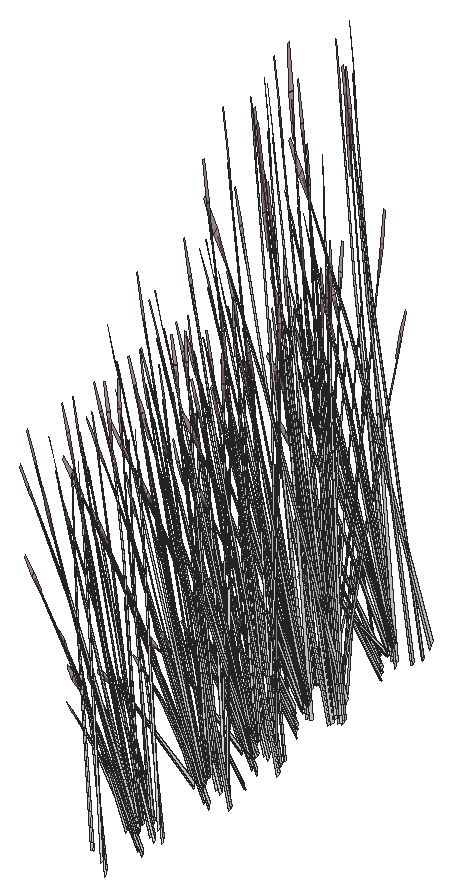
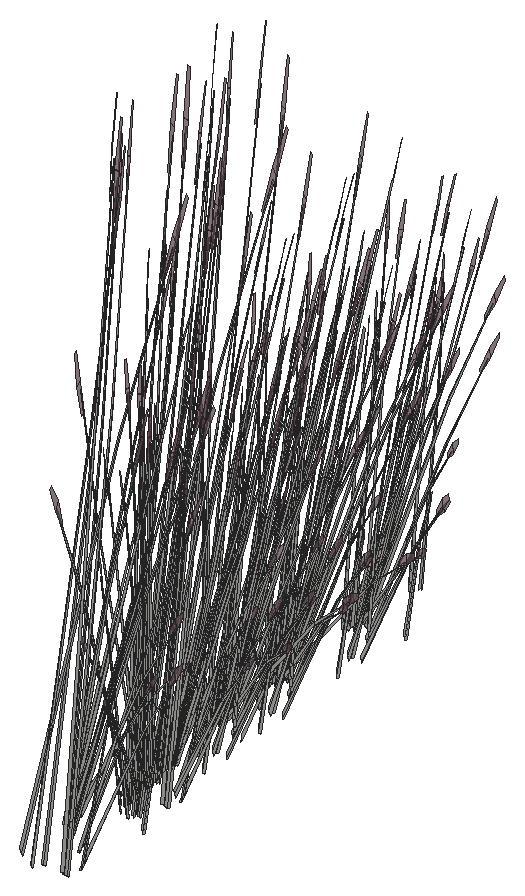
# SketchUp Ruby script. Lengths in inches.
U = 1.inch
M = Sketchup.active_model
def pt(a) = Geom::Point3d.new(a.map { |v| v * U })
def face(e, loops, mat)
  f = e.add_face(loops[0].map { |a| pt(a) })
  loops[1..].each { |l| e.add_face(l.map { |a| pt(a) }).erase! }
  f.material = f.back_material = mat if mat
  f
end
# faces: each face lists its corners as indices into pts; further lists are holes
def faces(e, pts, list, mat = nil) = list.each { |f| face(e, (f[0].is_a?(Array) ? f : [f]).map { |l| l.map { |i| pts[i] } }, mat) }
# xy, xz, yz: faces in a plane at the given z, y or x. An outline is a flat list of corners, or four numbers for a rectangle; further outlines are holes
def ring(l) = l.size == 4 ? [[l[0], l[1]], [l[2], l[1]], [l[2], l[3]], [l[0], l[3]]] : l.each_slice(2).to_a
def flat(e, list, mat, &to3) = list.each { |f| face(e, (f[0].is_a?(Array) ? f : [f]).map { |l| ring(l).map { |u, v| to3.(u, v) } }, mat) }
def xy(e, z, list, mat = nil) = flat(e, list, mat) { |x, y| [x, y, z] }
def xz(e, y, list, mat = nil) = flat(e, list, mat) { |x, z| [x, y, z] }
def yz(e, x, list, mat = nil) = flat(e, list, mat) { |y, z| [x, y, z] }
def lines(e, pts, list) = list.each { |a, b| e.add_line(pt(pts[a]), pt(pts[b])) }
# prism: a flat outline (further loops are holes) pulled along v
def prism(e, loops, v, mat = nil)
  f = face(e, loops, mat); d = Geom::Vector3d.new(v.map { |x| x * U })
  f.pushpull(f.normal.samedirection?(d) ? d.length : -d.length)
end
def box(e, o, s, mat = nil) = prism(e, [[o, [o[0] + s[0], o[1], o[2]], [o[0] + s[0], o[1] + s[1], o[2]], [o[0], o[1] + s[1], o[2]]]], [0, 0, s[2]], mat)
def at(x, y, z, deg = 0) = Geom::Transformation.translation(pt([x, y, z])) * Geom::Transformation.rotation(ORIGIN, Z_AXIS, deg.degrees)
def axes(o, x, y, z) = Geom::Transformation.new([*x, 0, *y, 0, *z, 0, *pt(o).to_a, 1])
def part(name) = M.definitions.add(name)
# library, detail: a bought-in or finely detailed component or shape, given as its bounding box
def library(name, o, s) = part(name).tap { |d| box(d.entities, o, s) }
def detail(e, o, s) = box(e.add_group.entities, o, s)
def put(e, d, t, mat = nil) = e.add_instance(d, t).tap { |i| i.material = mat if mat }
def group(e, t, mat = nil) = e.add_group.tap { |g| g.transformation = t; g.material = mat if mat }.entities
root = M.entities
M.materials.add("LightPink_Translucent").color = [144, 107, 117]
M.materials["LightPink_Translucent"].alpha = 0.75
c1 = part("blade")
p = [[2.15,0.21,22],[0,0.17,0],[0.09,0.45,0],[2.18,0.31,22],[2.29,0.31,22],[0.38,0.45,0],
  [2.48,0.24,33],[2.49,0.24,33],[2.48,0.22,33]]
faces(c1.entities,p,[[0,1,2,3],[4,5,2,3],[6,3,4,7],[8,0,3,6]])
c2 = part("seeds")
p = [[0.3,-0.1,1.38],[-0.01,-0.03,1.59],[-0.01,-0.03,0.03],[0.14,-0.07,-0.07],[0.29,-0.03,3],[0.15,0.01,3.11]]
faces(c2.entities,p,[[0,1,2,3],[1,0,4,5]],"LightPink_Translucent")
c3 = part("blade with seeds")
put(c3.entities,c1,at(0,0,0))
put(c3.entities,c2,axes([2.4,0.25,30.99],[1.5799,-0.05474,1.17369],[-0.12525,1.92788,0.29478],[-0.07173,-0.02425,1.56792]))
put(root,c3,axes([408.59,291.07,-7.78],[-0.44516,0.07768,-0.32977],[-0.11755,-0.44407,0.42575],[-0.12757,0.11927,0.81462]))
put(root,c3,axes([409.1875,295.16,-7.78],[-0.29098,-0.34031,-0.32977],[0.33226,-0.32215,0.42575],[-0.16881,-0.04902,0.81462]))
put(root,c3,axes([409.08,295.52,-9.59],[0.09985,0.15133,1.33163],[-0.23008,0.41134,-0.28638],[-0.23625,-0.09832,0.56934]))
put(root,c3,axes([409.49,295.39,-7.36],[-0.51122,-0.01309,-0.66157],[0.03434,-0.5511,0.07984],[-0.21658,-0.05816,0.93586]))
put(root,c3,axes([409.36,290.63,-8.39],[0.12773,-0.16701,1.59586],[0.32252,0.4508,0.12904],[-0.22121,0.20529,0.68222]))
put(root,c3,axes([408.35,292.39,-10.61],[0.0686,0.0543,1.6421],[0.11632,0.50315,-0.25086],[-0.15204,0.10729,0.2797]))
put(root,c3,axes([408.8,294.49,-7.62],[0.03791,0.05424,1.65179],[-0.18278,0.48761,-0.15608],[-0.18511,0.00353,0.29231]))
put(root,c3,axes([409.32,295.5,-7.64],[-0.37135,0.36005,-0.47583],[-0.32522,-0.38035,-0.36857],[-0.18868,-0.05478,0.91046]))
put(root,c3,axes([408.49,295.98,-9.42],[0.3265,-0.03889,1.06958],[-0.20711,0.3427,0.78586],[-0.16135,-0.05141,0.23558]))
put(root,c3,axes([409.52,295.12,-7.3125],[-0.02738,0.55277,-0.11324],[-0.51847,-0.01511,-0.62851],[-0.19968,-0.0384,0.95501]))
put(root,c3,axes([408.86,295.88,-8.39],[0.21212,-0.01231,1.59586],[-0.14072,0.53355,0.12904],[-0.3023,-0.033,0.68222]))
put(root,c3,axes([408.77,296.29,-7.59],[0.14449,-0.4956,0.447],[0.47502,0.16947,0.36857],[-0.1868,0.02978,0.92496]))
put(root,c3,axes([408.74,296.16,-7.6],[-0.18783,-0.37061,0.05988],[0.34252,-0.1814,0.47138],[-0.15099,0.03579,0.71878]))
put(root,c3,axes([408.73,296.54,-10.61],[0.01297,0.08566,1.6421],[-0.26146,0.44735,-0.25086],[-0.18572,-0.02255,0.2797]))
put(root,c3,axes([408.67,296.34,-7.78],[-0.42502,-0.15163,-0.32977],[0.12396,-0.44238,0.42575],[-0.17112,0.04056,0.81462]))
put(root,c3,axes([409.97,296.27,-8.89],[0.14537,-0.07863,1.64882],[0.05013,0.549,0.12904],[-0.31487,0.07285,0.5893]))
put(root,c3,axes([408.4,296.64,-7.61],[-0.08351,0.07057,1.62908],[0.0071,0.51561,-0.25764],[-0.19143,0.06705,0.13065]))
put(root,c3,axes([408.96,296.57,-7.64],[-0.13855,0.49442,-0.47583],[-0.47502,-0.16947,-0.36857],[-0.19125,0.04534,0.91046]))
put(root,c3,axes([408.94,296.14,-7.3125],[0.25732,0.49218,-0.11324],[-0.45669,0.24187,-0.62851],[-0.19245,0.06494,0.95501]))
put(root,c3,axes([408.89,297.52,-7.59],[-0.12683,-0.50025,0.447],[0.49754,-0.08682,0.36857],[-0.14663,0.11765,0.92496]))
put(root,c3,axes([408.95,296.82,-8.39],[0.17745,-0.11497,1.59586],[0.14939,0.53127,0.12904],[-0.27857,0.12007,0.68222]))
put(root,c3,axes([408.4,297.73,-9.59],[0.17773,0.04462,1.33163],[0.11455,0.45576,-0.28638],[-0.24142,0.08531,0.56934]))
put(root,c3,axes([407.48,297.16,-7.62],[0.06527,0.01458,1.65179],[0.20191,0.48025,-0.15608],[-0.1336,0.12605,0.29231]))
put(root,c3,axes([408.02,298.68,-9.42],[0.21313,-0.24635,1.06958],[0.0841,0.38999,0.78586],[-0.15402,0.06983,0.23558]))
put(root,c3,axes([408.83,297.62,-7.78],[-0.44516,0.07768,-0.32977],[-0.11755,-0.44407,0.42575],[-0.12757,0.11927,0.81462]))
put(root,c3,axes([409.6,297.18,-8.39],[0.12773,-0.16701,1.59586],[0.32252,0.4508,0.12904],[-0.22121,0.20529,0.68222]))
put(root,c3,axes([408.66,303.79,-8.39],[0.18996,0.09365,1.59586],[-0.39312,0.39287,0.12904],[-0.24502,-0.17723,0.68222]))
put(root,c3,axes([408.59,298.94,-10.61],[0.0686,0.0543,1.6421],[0.11632,0.50315,-0.25086],[-0.15204,0.10729,0.2797]))
put(root,c3,axes([408.62,302.93,-7.61],[-0.11004,-0.00384,1.62908],[-0.35032,0.38367,-0.25764],[-0.18692,-0.07839,0.13065]))
put(root,c3,axes([408.54,303.8,-7.26],[0.42234,-0.40113,0.50064],[0.36424,0.42599,0.4128],[-0.19815,-0.07399,1.03595]))
put(root,c3,axes([408.73,303.79,-7.6],[0.02575,-0.41332,0.05988],[0.38885,0.01133,0.47138],[-0.14895,-0.04325,0.71878]))
put(root,c3,axes([408.58,303.93,-7.78],[-0.29098,-0.34031,-0.32977],[0.33226,-0.32215,0.42575],[-0.16881,-0.04902,0.81462]))
put(root,c3,axes([408.48,304.29,-9.59],[0.09985,0.15133,1.33163],[-0.23008,0.41134,-0.28638],[-0.23625,-0.09832,0.56934]))
put(root,c3,axes([408.89,304.15,-7.36],[-0.51122,-0.01309,-0.66157],[0.03434,-0.5511,0.07984],[-0.21658,-0.05816,0.93586]))
put(root,c3,axes([408.2,303.25,-7.62],[0.03791,0.05424,1.65179],[-0.18278,0.48761,-0.15608],[-0.18511,0.00353,0.29231]))
put(root,c3,axes([408.72,304.26,-7.64],[-0.37135,0.36005,-0.47583],[-0.32522,-0.38035,-0.36857],[-0.18868,-0.05478,0.91046]))
put(root,c3,axes([407.88,304.74,-9.42],[0.3265,-0.03889,1.06958],[-0.20711,0.3427,0.78586],[-0.16135,-0.05141,0.23558]))
put(root,c3,axes([408.92,303.89,-7.3125],[-0.02738,0.55277,-0.11324],[-0.51847,-0.01511,-0.62851],[-0.19968,-0.0384,0.95501]))
put(root,c3,axes([408.26,304.65,-8.39],[0.21212,-0.01231,1.59586],[-0.14072,0.53355,0.12904],[-0.3023,-0.033,0.68222]))
put(root,c3,axes([409.83,306.08,-10.08],[-0.53199,-0.08911,-0.58063],[0.11226,-0.54969,-0.15239],[-0.15876,-0.06661,1.28164]))
put(root,c3,axes([408.17,305.05,-7.59],[0.14449,-0.4956,0.447],[0.47502,0.16947,0.36857],[-0.1868,0.02978,0.92496]))
put(root,c3,axes([408.13,304.92,-7.6],[-0.18783,-0.37061,0.05988],[0.34252,-0.1814,0.47138],[-0.15099,0.03579,0.71878]))
put(root,c3,axes([408.12,305.3,-10.61],[0.01297,0.08566,1.6421],[-0.26146,0.44735,-0.25086],[-0.18572,-0.02255,0.2797]))
put(root,c3,axes([408.07,305.11,-7.78],[-0.42502,-0.15163,-0.32977],[0.12396,-0.44238,0.42575],[-0.17112,0.04056,0.81462]))
put(root,c3,axes([408.52,305.06,-7.3],[0.42502,0.15163,0.32977],[-0.12396,0.44238,-0.42575],[-0.17112,0.04056,0.81462]))
put(root,c3,axes([409.36,305.03,-8.89],[0.14537,-0.07863,1.64882],[0.05013,0.549,0.12904],[-0.31487,0.07285,0.5893]))
put(root,c3,axes([409.33,309.79,-7.36],[-0.43608,-0.26272,-0.66157],[0.30991,-0.46038,0.07984],[-0.158,-0.15687,0.93586]))
put(root,c3,axes([407.8,305.4,-7.61],[-0.08351,0.07057,1.62908],[0.0071,0.51561,-0.25764],[-0.19143,0.06705,0.13065]))
put(root,c3,axes([408.36,305.33,-7.64],[-0.13855,0.49442,-0.47583],[-0.47502,-0.16947,-0.36857],[-0.19125,0.04534,0.91046]))
put(root,c3,axes([408.34,304.91,-7.3125],[0.25732,0.49218,-0.11324],[-0.45669,0.24187,-0.62851],[-0.19245,0.06494,0.95501]))
put(root,c3,axes([408.47,309.36,-10.61],[-0.04954,0.0716,1.6421],[-0.50062,0.15438,-0.25086],[-0.12094,-0.14044,0.2797]))
put(root,c3,axes([408.21,310.08,-8.39],[0.18996,0.09365,1.59586],[-0.39312,0.39287,0.12904],[-0.24502,-0.17723,0.68222]))
put(root,c3,axes([409.125,309.8,-7.64],[-0.50465,0.12921,-0.47583],[-0.08828,-0.48932,-0.36857],[-0.13555,-0.14022,0.91046]))
put(root,c3,axes([409.48,309.37,-6.94],[-0.34131,0.52108,-0.12682],[-0.49429,-0.3002,-0.70393],[-0.17182,-0.14722,1.06961]))
put(root,c3,axes([408.28,306.29,-7.59],[-0.12683,-0.50025,0.447],[0.49754,-0.08682,0.36857],[-0.14663,0.11765,0.92496]))
put(root,c3,axes([408.18,306.19,-7.6],[-0.35109,-0.22859,0.05988],[0.2044,-0.32553,0.47138],[-0.11256,0.10524,0.71878]))
put(root,c3,axes([408.34,305.59,-8.39],[0.17745,-0.11497,1.59586],[0.14939,0.53127,0.12904],[-0.27857,0.12007,0.68222]))
put(root,c3,axes([408.17,309.22,-7.61],[-0.11004,-0.00384,1.62908],[-0.35032,0.38367,-0.25764],[-0.18692,-0.07839,0.13065]))
put(root,c3,axes([407.79,306.49,-9.59],[0.17773,0.04462,1.33163],[0.11455,0.45576,-0.28638],[-0.24142,0.08531,0.56934]))
put(root,c3,axes([408.09,310.09,-7.26],[0.42234,-0.40113,0.50064],[0.36424,0.42599,0.4128],[-0.19815,-0.07399,1.03595]))
put(root,c3,axes([406.875,305.92,-7.62],[0.06527,0.01458,1.65179],[0.20191,0.48025,-0.15608],[-0.1336,0.12605,0.29231]))
put(root,c3,axes([407.42,307.45,-9.42],[0.21313,-0.24635,1.06958],[0.0841,0.38999,0.78586],[-0.15402,0.06983,0.23558]))
put(root,c3,axes([408.23,306.38,-7.78],[-0.44516,0.07768,-0.32977],[-0.11755,-0.44407,0.42575],[-0.12757,0.11927,0.81462]))
put(root,c3,axes([408.28,310.08,-7.6],[0.02575,-0.41332,0.05988],[0.38885,0.01133,0.47138],[-0.14895,-0.04325,0.71878]))
put(root,c3,axes([408.13,310.21,-7.78],[-0.29098,-0.34031,-0.32977],[0.33226,-0.32215,0.42575],[-0.16881,-0.04902,0.81462]))
put(root,c3,axes([408.03,310.57,-9.59],[0.09985,0.15133,1.33163],[-0.23008,0.41134,-0.28638],[-0.23625,-0.09832,0.56934]))
put(root,c3,axes([408.4375,310.44,-7.36],[-0.51122,-0.01309,-0.66157],[0.03434,-0.5511,0.07984],[-0.21658,-0.05816,0.93586]))
put(root,c3,axes([408.99,305.94,-8.39],[0.12773,-0.16701,1.59586],[0.32252,0.4508,0.12904],[-0.22121,0.20529,0.68222]))
put(root,c3,axes([408.59,306.43,-7.64],[0.13138,0.49631,-0.47583],[-0.49754,0.08682,-0.36857],[-0.14258,0.13331,0.91046]))
put(root,c3,axes([407.75,309.54,-7.62],[0.03791,0.05424,1.65179],[-0.18278,0.48761,-0.15608],[-0.18511,0.00353,0.29231]))
put(root,c3,axes([407.98,307.7,-10.61],[0.0686,0.0543,1.6421],[0.11632,0.50315,-0.25086],[-0.15204,0.10729,0.2797]))
put(root,c3,axes([408.27,310.55,-7.64],[-0.37135,0.36005,-0.47583],[-0.32522,-0.38035,-0.36857],[-0.18868,-0.05478,0.91046]))
put(root,c3,axes([408.54,310.39,-7.3],[0.29098,0.34031,0.32977],[-0.33226,0.32215,-0.42575],[-0.16881,-0.04902,0.81462]))
put(root,c3,axes([407.43,311.03,-9.42],[0.3265,-0.03889,1.06958],[-0.20711,0.3427,0.78586],[-0.16135,-0.05141,0.23558]))
put(root,c3,axes([408.46,310.17,-7.3125],[-0.02738,0.55277,-0.11324],[-0.51847,-0.01511,-0.62851],[-0.19968,-0.0384,0.95501]))
put(root,c3,axes([408.9,306.36,-8.39],[0.09522,-0.18683,1.59586],[0.39947,0.38663,0.12904],[-0.18021,0.24097,0.68222]))
put(root,c3,axes([407.82,307.33,-7.61],[-0.01271,0.10756,1.62908],[0.36076,0.37419,-0.25764],[-0.09444,0.17695,0.13065]))
put(root,c3,axes([409.38,312.37,-10.08],[-0.53199,-0.08911,-0.58063],[0.11226,-0.54969,-0.15239],[-0.15876,-0.06661,1.28164]))
put(root,c3,axes([407.72,311.34,-7.59],[0.14449,-0.4956,0.447],[0.47502,0.16947,0.36857],[-0.1868,0.02978,0.92496]))
put(root,c3,axes([407.68,311.21,-7.6],[-0.18783,-0.37061,0.05988],[0.34252,-0.1814,0.47138],[-0.15099,0.03579,0.71878]))
put(root,c3,axes([407.67,311.59,-10.61],[0.01297,0.08566,1.6421],[-0.26146,0.44735,-0.25086],[-0.18572,-0.02255,0.2797]))
put(root,c3,axes([408.68,313.41,-10.12],[-0.47863,-0.27177,-0.46235],[0.28609,-0.48733,0],[-0.10901,-0.0619,1.46668]))
put(root,c3,axes([407.62,311.39,-7.78],[-0.42502,-0.15163,-0.32977],[0.12396,-0.44238,0.42575],[-0.17112,0.04056,0.81462]))
put(root,c3,axes([408.07,311.35,-7.3],[0.42502,0.15163,0.32977],[-0.12396,0.44238,-0.42575],[-0.17112,0.04056,0.81462]))
put(root,c3,axes([408.91,311.32,-8.89],[0.14537,-0.07863,1.64882],[0.05013,0.549,0.12904],[-0.31487,0.07285,0.5893]))
put(root,c3,axes([407.35,311.6875,-7.61],[-0.08351,0.07057,1.62908],[0.0071,0.51561,-0.25764],[-0.19143,0.06705,0.13065]))
put(root,c3,axes([407.91,311.62,-7.64],[-0.13855,0.49442,-0.47583],[-0.47502,-0.16947,-0.36857],[-0.19125,0.04534,0.91046]))
put(root,c3,axes([407.89,311.2,-7.3125],[0.25732,0.49218,-0.11324],[-0.45669,0.24187,-0.62851],[-0.19245,0.06494,0.95501]))
put(root,c3,axes([408.97,313.73,-9.79],[-0.31974,0.54466,0],[-0.53494,-0.30375,-0.48057],[-0.12184,-0.06918,1.52448]))
put(root,c3,axes([407.08,318.05,-8.39],[0.1169,0.17452,1.59586],[-0.54019,0.14692,0.12904],[-0.12209,-0.27397,0.68222]))
put(root,c3,axes([406.93,317.59,-9.59],[-0.03097,0.17781,1.33163],[-0.45273,0.14885,-0.28638],[-0.10583,-0.22982,0.56934]))
put(root,c3,axes([407.83,312.57,-7.59],[-0.12683,-0.50025,0.447],[0.49754,-0.08682,0.36857],[-0.14663,0.11765,0.92496]))
put(root,c3,axes([407.73,312.48,-7.6],[-0.35109,-0.22859,0.05988],[0.2044,-0.32553,0.47138],[-0.11256,0.10524,0.71878]))
put(root,c3,axes([407.89,311.875,-8.39],[0.17745,-0.11497,1.59586],[0.14939,0.53127,0.12904],[-0.27857,0.12007,0.68222]))
put(root,c3,axes([407.34,312.78,-9.59],[0.17773,0.04462,1.33163],[0.11455,0.45576,-0.28638],[-0.24142,0.08531,0.56934]))
put(root,c3,axes([407.4375,316.65,-7.62],[-0.00954,0.06515,1.65179],[-0.47055,0.23645,-0.15608],[-0.13847,-0.12087,0.29231]))
put(root,c3,axes([406.42,312.21,-7.62],[0.06527,0.01458,1.65179],[0.20191,0.48025,-0.15608],[-0.1336,0.12605,0.29231]))
put(root,c3,axes([406.97,313.74,-9.42],[0.21313,-0.24635,1.06958],[0.0841,0.38999,0.78586],[-0.15402,0.06983,0.23558]))
put(root,c3,axes([407.34,317.8,-7.26],[0.56969,-0.13971,0.50064],[0.09887,0.54803,0.4128],[-0.13398,-0.16152,1.03595]))
put(root,c3,axes([407.77,312.67,-7.78],[-0.44516,0.07768,-0.32977],[-0.11755,-0.44407,0.42575],[-0.12757,0.11927,0.81462]))
put(root,c3,axes([406.78,317.31,-9.42],[0.26677,0.18918,1.06958],[-0.38851,0.11372,0.78586],[-0.08313,-0.14539,0.23558]))
put(root,c3,axes([407.42,318.31,-7.36],[-0.43608,-0.26272,-0.66157],[0.30991,-0.46038,0.07984],[-0.158,-0.15687,0.93586]))
put(root,c3,axes([407.27,317.96,-7.78],[-0.07899,-0.43781,-0.32977],[0.45153,-0.11561,0.42575],[-0.12128,-0.12546,0.81462]))
put(root,c3,axes([407.47,317.92,-7.6],[0.23243,-0.34529,0.05988],[0.331,0.20103,0.47138],[-0.10701,-0.1107,0.71878]))
put(root,c3,axes([406.57,317.875,-10.61],[-0.04954,0.0716,1.6421],[-0.50062,0.15438,-0.25086],[-0.12094,-0.14044,0.2797]))
put(root,c3,axes([407.91,312.37,-7.3125],[0.47307,0.29971,-0.11324],[-0.27254,0.43404,-0.62851],[-0.13365,0.15087,0.95501]))
put(root,c3,axes([408.54,312.23,-8.39],[0.12773,-0.16701,1.59586],[0.32252,0.4508,0.12904],[-0.22121,0.20529,0.68222]))
put(root,c3,axes([407.22,318.32,-7.64],[-0.50465,0.12921,-0.47583],[-0.08828,-0.48932,-0.36857],[-0.13555,-0.14022,0.91046]))
put(root,c3,axes([408.14,312.72,-7.64],[0.13138,0.49631,-0.47583],[-0.49754,0.08682,-0.36857],[-0.14258,0.13331,0.91046]))
put(root,c3,axes([407.57,317.88,-6.94],[-0.34131,0.52108,-0.12682],[-0.49429,-0.3002,-0.70393],[-0.17182,-0.14722,1.06961]))
put(root,c3,axes([407.53,313.99,-10.61],[0.0686,0.0543,1.6421],[0.11632,0.50315,-0.25086],[-0.15204,0.10729,0.2797]))
put(root,c3,axes([408.47,321.28,-8.9],[0.44194,0.21918,1.40854],[-0.43295,0.47219,0.557],[-0.19393,-0.27986,1.18082]))
put(root,c3,axes([407.54,318.32,-7.3],[0.07899,0.43781,0.32977],[-0.45153,0.11561,-0.42575],[-0.12128,-0.12546,0.81462]))
put(root,c3,axes([406.18,318.6,-7.26],[0.42234,-0.40113,0.50064],[0.36424,0.42599,0.4128],[-0.19815,-0.07399,1.03595]))
put(root,c3,axes([408.45,312.64,-8.39],[0.09522,-0.18683,1.59586],[0.39947,0.38663,0.12904],[-0.18021,0.24097,0.68222]))
put(root,c3,axes([407.36,313.61,-7.61],[-0.01271,0.10756,1.62908],[0.36076,0.37419,-0.25764],[-0.09444,0.17695,0.13065]))
put(root,c3,axes([406.375,318.6,-7.6],[0.02575,-0.41332,0.05988],[0.38885,0.01133,0.47138],[-0.14895,-0.04325,0.71878]))
put(root,c3,axes([406.23,318.73,-7.78],[-0.29098,-0.34031,-0.32977],[0.33226,-0.32215,0.42575],[-0.16881,-0.04902,0.81462]))
put(root,c3,axes([406.26,318.15,-10.02],[-0.14753,0.44383,-0.03625],[-0.45406,-0.13653,-0.16435],[-0.06894,-0.07259,0.54209]))
put(root,c3,axes([406.01,320.18,-9.79],[-0.63949,0,0],[0,-0.60749,-0.48057],[0,-0.13836,1.52448]))
put(root,c3,axes([406.51,320.02,-9.83],[-0.47569,0.45698,0.2864],[-0.47598,-0.45217,-0.33981],[-0.01661,-0.12977,1.53541]))
put(root,c3,axes([407.8,320.97,-9.73],[0.13555,-0.64407,-0.21817],[0.64269,0.11227,0.47743],[-0.1123,-0.08895,1.45677]))
put(root,c3,axes([406.64,318.91,-7.3],[0.29098,0.34031,0.32977],[-0.33226,0.32215,-0.42575],[-0.16881,-0.04902,0.81462]))
put(root,c3,axes([405.53,319.55,-9.42],[0.3265,-0.03889,1.06958],[-0.20711,0.3427,0.78586],[-0.16135,-0.05141,0.23558]))
put(root,c3,axes([406.56,318.69,-7.3125],[-0.02738,0.55277,-0.11324],[-0.51847,-0.01511,-0.62851],[-0.19968,-0.0384,0.95501]))
put(root,c3,axes([407.75,320.71,-9.94],[-0.30722,-0.45622,-0.41661],[0.46535,-0.32126,0.2005],[-0.09942,-0.05645,1.33761]))
put(root,c3,axes([407.47,320.88,-10.08],[-0.53199,-0.08911,-0.58063],[0.11226,-0.54969,-0.15239],[-0.15876,-0.06661,1.28164]))
put(root,c3,axes([405.77,319.73,-7.6],[-0.18783,-0.37061,0.05988],[0.34252,-0.1814,0.47138],[-0.15099,0.03579,0.71878]))
put(root,c3,axes([406.91,321.72,-10.11],[-0.12013,-0.47362,-0.28847],[0.47712,-0.13449,0.28847],[-0.09619,-0.05462,1.29413]))
put(root,c3,axes([406.78,321.92,-10.12],[-0.47863,-0.27177,-0.46235],[0.28609,-0.48733,0],[-0.10901,-0.0619,1.46668]))
put(root,c3,axes([408.08,320.96,-9.52],[-0.51635,0.36087,-0.27094],[-0.34336,-0.5099,-0.46562],[-0.1274,-0.05178,1.4872]))
put(root,c3,axes([408.03,321.12,-9.5625],[-0.09866,0.48509,0.13483],[-0.48202,-0.0842,-0.38503],[-0.08772,-0.04981,1.18024]))
put(root,c3,axes([406.16,319.86,-7.3],[0.42502,0.15163,0.32977],[-0.12396,0.44238,-0.42575],[-0.17112,0.04056,0.81462]))
put(root,c3,axes([408.66,321.13,-9.7],[-0.49938,-0.43748,-0.23459],[0.42021,-0.49126,0.51337],[-0.13447,0.05118,1.56642]))
put(root,c3,axes([407.34,321.97,-9.69],[0.47863,0.27177,0.46235],[-0.28609,0.48733,0],[-0.10901,-0.0619,1.46668]))
put(root,c3,axes([407.07,322.25,-9.79],[-0.31974,0.54466,0],[-0.53494,-0.30375,-0.48057],[-0.12184,-0.06918,1.52448]))
put(root,c3,axes([408.41,321.04,-9.94],[-0.55535,0.03355,-0.41661],[-0.05022,-0.55698,0.2005],[-0.09942,0.05645,1.33761]))
put(root,c3,axes([405.93,321.09,-7.59],[-0.12683,-0.50025,0.447],[0.49754,-0.08682,0.36857],[-0.14663,0.11765,0.92496]))
put(root,c3,axes([405.83,321,-7.6],[-0.35109,-0.22859,0.05988],[0.2044,-0.32553,0.47138],[-0.11256,0.10524,0.71878]))
put(root,c3,axes([406.23,320.93,-7.3],[0.44516,-0.07768,0.32977],[0.11755,0.44407,-0.42575],[-0.12757,0.11927,0.81462]))
put(root,c3,axes([405.87,321.1875,-7.78],[-0.44516,0.07768,-0.32977],[-0.11755,-0.44407,0.42575],[-0.12757,0.11927,0.81462]))
put(root,c3,axes([405.22,322.1875,-6.74],[0.45129,0.14509,-0.06041],[-0.13882,0.44656,-0.27392],[-0.07381,0.0678,0.90349]))
put(root,c3,axes([408.42,321.36,-10.08],[-0.34446,0.40855,-0.58063],[-0.42791,-0.37046,-0.15239],[-0.13803,0.10191,1.28164]))
put(root,c3,axes([406,320.88,-7.3125],[0.47307,0.29971,-0.11324],[-0.27254,0.43404,-0.62851],[-0.13365,0.15087,0.95501]))
put(root,c3,axes([406.53,328.95,-8.39],[0.1169,0.17452,1.59586],[-0.54019,0.14692,0.12904],[-0.12209,-0.27397,0.68222]))
put(root,c3,axes([406.64,320.75,-8.39],[0.12773,-0.16701,1.59586],[0.32252,0.4508,0.12904],[-0.22121,0.20529,0.68222]))
put(root,c3,axes([406.23,321.24,-7.64],[0.13138,0.49631,-0.47583],[-0.49754,0.08682,-0.36857],[-0.14258,0.13331,0.91046]))
put(root,c3,axes([407.43,327.79,-7.61],[-0.07822,-0.07621,1.62908],[-0.52201,0.04832,-0.25764],[-0.08331,-0.18228,0.13065]))
put(root,c3,axes([406.52,322.07,-7.6],[-0.42027,-0.02533,0.05988],[0.01152,-0.38243,0.47138],[-0.04398,0.14649,0.71878]))
put(root,c3,axes([406.39,328.49,-9.59],[-0.03097,0.17781,1.33163],[-0.45273,0.14885,-0.28638],[-0.10583,-0.22982,0.56934]))
put(root,c3,axes([405.625,322.51,-10.61],[0.0686,0.0543,1.6421],[0.11632,0.50315,-0.25086],[-0.15204,0.10729,0.2797]))
put(root,c3,axes([406.65,322.1,-7.59],[-0.36417,-0.37086,0.447],[0.38674,-0.31985,0.36857],[-0.06718,0.174,0.92496]))
put(root,c3,axes([406.54,321.16,-8.39],[0.09522,-0.18683,1.59586],[0.39947,0.38663,0.12904],[-0.18021,0.24097,0.68222]))
put(root,c3,axes([406.89,327.54,-7.62],[-0.00954,0.06515,1.65179],[-0.47055,0.23645,-0.15608],[-0.13847,-0.12087,0.29231]))
put(root,c3,axes([406.65,322.22,-7.78],[-0.34603,0.28618,-0.32977],[-0.32756,-0.32677,0.42575],[-0.04984,0.16603,0.81462]))
put(root,c3,axes([405.46,322.13,-7.61],[-0.01271,0.10756,1.62908],[0.36076,0.37419,-0.25764],[-0.09444,0.17695,0.13065]))
put(root,c3,axes([406.79,328.7,-7.26],[0.56969,-0.13971,0.50064],[0.09887,0.54803,0.4128],[-0.13398,-0.16152,1.03595]))
put(root,c3,axes([406.87,323.33,-9.42],[-0.01324,-0.32319,1.06958],[0.33072,0.23052,0.78586],[-0.06504,0.15405,0.23558]))
put(root,c3,axes([406.23,328.2,-9.42],[0.26677,0.18918,1.06958],[-0.38851,0.11372,0.78586],[-0.08313,-0.14539,0.23558]))
put(root,c3,axes([406.875,329.21,-7.36],[-0.43608,-0.26272,-0.66157],[0.30991,-0.46038,0.07984],[-0.158,-0.15687,0.93586]))
put(root,c3,axes([406.72,328.86,-7.78],[-0.07899,-0.43781,-0.32977],[0.45153,-0.11561,0.42575],[-0.12128,-0.12546,0.81462]))
put(root,c3,axes([406.92,328.82,-7.6],[0.23243,-0.34529,0.05988],[0.331,0.20103,0.47138],[-0.10701,-0.1107,0.71878]))
put(root,c3,axes([406.02,328.77,-10.61],[-0.04954,0.0716,1.6421],[-0.50062,0.15438,-0.25086],[-0.12094,-0.14044,0.2797]))
put(root,c3,axes([406.88,321.91,-7.03],[-0.01331,0.50278,-0.73435],[-0.56035,-0.03377,0.08862],[-0.05914,0.213,1.03881]))
put(root,c3,axes([405.42,323.23,-7.62],[0.05802,-0.03282,1.65179],[0.47954,0.21828,-0.15608],[-0.01127,0.18175,0.29231]))
put(root,c3,axes([406.67,329.22,-7.64],[-0.50465,0.12921,-0.47583],[-0.08828,-0.48932,-0.36857],[-0.13555,-0.14022,0.91046]))
put(root,c3,axes([407.02,328.78,-6.94],[-0.34131,0.52108,-0.12682],[-0.49429,-0.3002,-0.70393],[-0.17182,-0.14722,1.06961]))
put(root,c3,axes([406.49,323.04,-9.59],[0.16138,-0.08575,1.33163],[0.39845,0.25854,-0.28638],[-0.1186,0.22371,0.56934]))
put(root,c3,axes([407.92,332.18,-8.9],[0.44194,0.21918,1.40854],[-0.43295,0.47219,0.557],[-0.19393,-0.27986,1.18082]))
put(root,c3,axes([406.99,329.22,-7.3],[0.07899,0.43781,0.32977],[-0.45153,0.11561,-0.42575],[-0.12128,-0.12546,0.81462]))
put(root,c3,axes([405.61,330.66,-10.12],[0,-0.54355,-0.46235],[0.57217,0,0],[0,-0.1238,1.46668]))
put(root,c3,axes([406.69,322.62,-8.87],[0.01124,-0.2806,1.43727],[0.50537,0.14821,0.19862],[-0.04379,0.29905,0.67868]))
put(root,c3,axes([405.83,329.5,-7.6],[0.02575,-0.41332,0.05988],[0.38885,0.01133,0.47138],[-0.14895,-0.04325,0.71878]))
put(root,c3,axes([405.71,329.05,-10.02],[-0.14753,0.44383,-0.03625],[-0.45406,-0.13653,-0.16435],[-0.06894,-0.07259,0.54209]))
put(root,c3,axes([407.1,331.29,-9.52],[-0.57594,-0.25935,-0.27094],[0.27732,-0.5474,-0.46562],[-0.0181,-0.1344,1.4872]))
put(root,c3,axes([405.46,331.08,-9.79],[-0.63949,0,0],[0,-0.60749,-0.48057],[0,-0.13836,1.52448]))
put(root,c3,axes([405.96,330.92,-9.83],[-0.47569,0.45698,0.2864],[-0.47598,-0.45217,-0.33981],[-0.01661,-0.12977,1.53541]))
put(root,c3,axes([407.25,331.87,-9.73],[0.13555,-0.64407,-0.21817],[0.64269,0.11227,0.47743],[-0.1123,-0.08895,1.45677]))
put(root,c3,axes([406.09,329.81,-7.3],[0.29098,0.34031,0.32977],[-0.33226,0.32215,-0.42575],[-0.16881,-0.04902,0.81462]))
